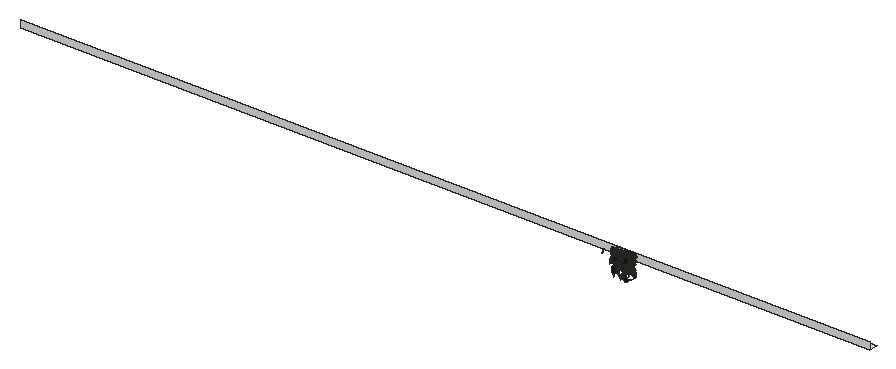
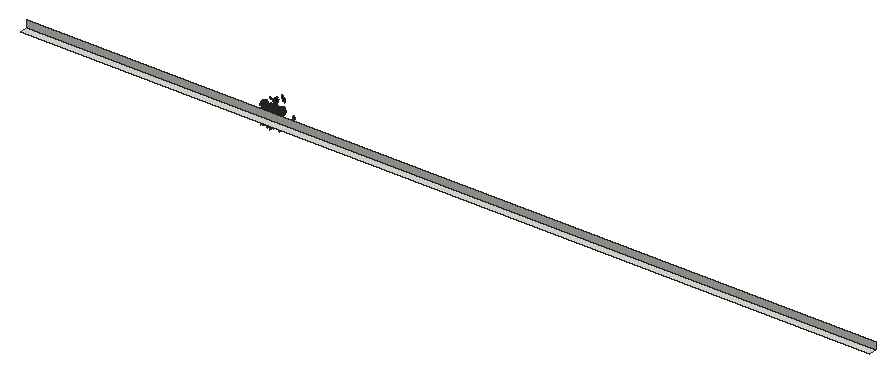
# SketchUp Ruby script. Lengths in inches.
U = 1.inch
M = Sketchup.active_model
def pt(a) = Geom::Point3d.new(a.map { |v| v * U })
def face(e, loops, mat)
  f = e.add_face(loops[0].map { |a| pt(a) })
  loops[1..].each { |l| e.add_face(l.map { |a| pt(a) }).erase! }
  f.material = f.back_material = mat if mat
  f
end
# faces: each face lists its corners as indices into pts; further lists are holes
def faces(e, pts, list, mat = nil) = list.each { |f| face(e, (f[0].is_a?(Array) ? f : [f]).map { |l| l.map { |i| pts[i] } }, mat) }
# xy, xz, yz: faces in a plane at the given z, y or x. An outline is a flat list of corners, or four numbers for a rectangle; further outlines are holes
def ring(l) = l.size == 4 ? [[l[0], l[1]], [l[2], l[1]], [l[2], l[3]], [l[0], l[3]]] : l.each_slice(2).to_a
def flat(e, list, mat, &to3) = list.each { |f| face(e, (f[0].is_a?(Array) ? f : [f]).map { |l| ring(l).map { |u, v| to3.(u, v) } }, mat) }
def xy(e, z, list, mat = nil) = flat(e, list, mat) { |x, y| [x, y, z] }
def xz(e, y, list, mat = nil) = flat(e, list, mat) { |x, z| [x, y, z] }
def yz(e, x, list, mat = nil) = flat(e, list, mat) { |y, z| [x, y, z] }
def lines(e, pts, list) = list.each { |a, b| e.add_line(pt(pts[a]), pt(pts[b])) }
# prism: a flat outline (further loops are holes) pulled along v
def prism(e, loops, v, mat = nil)
  f = face(e, loops, mat); d = Geom::Vector3d.new(v.map { |x| x * U })
  f.pushpull(f.normal.samedirection?(d) ? d.length : -d.length)
end
def box(e, o, s, mat = nil) = prism(e, [[o, [o[0] + s[0], o[1], o[2]], [o[0] + s[0], o[1] + s[1], o[2]], [o[0], o[1] + s[1], o[2]]]], [0, 0, s[2]], mat)
def at(x, y, z, deg = 0) = Geom::Transformation.translation(pt([x, y, z])) * Geom::Transformation.rotation(ORIGIN, Z_AXIS, deg.degrees)
def axes(o, x, y, z) = Geom::Transformation.new([*x, 0, *y, 0, *z, 0, *pt(o).to_a, 1])
def part(name) = M.definitions.add(name)
# library, detail: a bought-in or finely detailed component or shape, given as its bounding box
def library(name, o, s) = part(name).tap { |d| box(d.entities, o, s) }
def detail(e, o, s) = box(e.add_group.entities, o, s)
def put(e, d, t, mat = nil) = e.add_instance(d, t).tap { |i| i.material = mat if mat }
def group(e, t, mat = nil) = e.add_group.tap { |g| g.transformation = t; g.material = mat if mat }.entities
root = M.entities
M.materials.add("efeu1").color = [18, 25, 13]
M.materials.add("efeu2").color = [43, 57, 29]
c1 = part("ivyleaf_10")
p = [[0,0.5,-0.03],[-0.0625,2.02,-0.43],[-0.19,2.01,-0.46],[-0.54,1.05,-0.29],[-0.52,0.625,-0.18],[-0.83,0.76,-0.28],
  [-1.16,0.64,-0.33],[-1.15,0.33,-0.24],[-0.77,-0.39,0.02],[-0.3,-0.51,0.16],[0.04,-0.48,0.23],[-0.02,2.01,-0.4375],
  [-0.06,2.01,-0.43],[0.04,-0.49,0.23],[0.67,-0.49,0.14],[1.38,0.36,-0.2],[1.375,0.51,-0.24],[0.81,0.65,-0.19],
  [0.62,0.59,-0.15],[0.6,1.09,-0.28],[0.5,1.23,-0.31]]
faces(c1.entities,p,[[0,1,2,3,4,5,6,7,8,9,10],[11,12,0,13,14,15,16,17,18,19,20]],"efeu2")
c2 = part("ivyleaf_9")
p = [[1.54,2.16,1.25],[1.36,2.04,1.19],[-0.21,0.99,0.68],[-0.71,1.11,0.82],[-0.85,0.86,0.67],[-0.8,0.17,0.21],
  [-0.9,-0.01,0.1],[-0.67,-0.16,-0.02],[-0.08,-0.08,-0.05],[-0.03,-0.6,-0.4],[0.65,-0.88,-0.66],[0.83,-0.6,-0.49],
  [1.29,-0.42,-0.43],[1.8125,-0.07,-0.26],[1.21,0.44,0.15]]
faces(c2.entities,p,[[0,1,2,3,4,5,6,7,8,9,10,11,12,13,14]],"efeu1")
xy(root,168.16,[[244.16,136.53,244.11,139.97,600.44,145.72,600.49,142.28]])
p = [[244.16,136.53,171.1],[244.16,136.53,168.16],[600.49,142.28,168.16],[600.49,142.28,171.1]]
faces(root,p,[[0,1,2,3]])
put(root,c1,axes([491.37,136.93,169.94],[0.20074,-0.58166,-0.17189],[-0.07454,0.15603,-0.61504],[0.60193,0.2133,-0.01884]))
put(root,c1,axes([494.35,138.04,166.5],[-0.38169,-0.3296,0.38813],[-0.23509,-0.31621,-0.49971],[0.45167,-0.44311,0.0679]))
put(root,c1,axes([494.3,137.58,168],[0.18373,-0.60834,0.06607],[0.02662,-0.06098,-0.63543],[0.61134,0.18548,0.00781]))
put(root,c1,axes([494.72,137.03,171.04],[-0.16372,0.54731,0.35458],[-0.09874,0.34056,-0.57127],[-0.64461,-0.19117,-0.00256]))
put(root,c1,axes([495.41,137.17,171.99],[-0.50295,0.27441,0.28094],[-0.23738,0.15124,-0.57268],[-0.31286,-0.55589,-0.01712]))
put(root,c1,axes([495.4,138.16,164.79],[-0.06945,-0.30835,0.55556],[0.2111,-0.53832,-0.27239],[0.5993,0.15389,0.16033]))
put(root,c1,axes([495.74,137.63,167.37],[-0.02299,0.08652,0.64605],[-0.24024,-0.60207,0.07208],[0.60593,-0.23542,0.05309]))
put(root,c1,axes([495.42,137.59,171.71],[0.40154,0.35078,0.36417],[0.24129,0.27573,-0.53165],[-0.44435,0.46672,0.04039]))
put(root,c1,axes([495.91,137.89,166.02],[-0.33828,0.54486,-0.11963],[-0.06404,0.10105,0.64133],[0.55415,0.34429,0.00109]))
put(root,c1,axes([495.81,138.47,171.13],[0.42104,0.45198,-0.16049],[-0.13431,-0.09391,-0.61682],[-0.46044,0.44069,0.03316]))
put(root,c1,axes([495.91,138.46,171.92],[-0.42511,-0.46934,-0.09728],[0.07791,0.06064,-0.63302],[0.47294,-0.43186,0.01684]))
put(root,c1,axes([496.16,136.59,170.65],[-0.30939,0.56323,-0.31644],[-0.21372,0.24187,0.63946],[0.60966,0.37062,0.06358]))
put(root,c1,axes([495.99,137.91,167.24],[-0.27662,-0.55222,-0.22368],[0.11697,0.19147,-0.61738],[0.5842,-0.29982,0.0177]))
put(root,c1,axes([496.46,136.32,171.12],[0.49785,0.21772,0.48822],[-0.49567,-0.06182,0.53302],[0.20018,-0.69455,0.1056]))
put(root,c1,axes([496.28,138.06,165.92],[-0.42104,-0.49881,-0.03379],[0.02216,0.02551,-0.65276],[0.49947,-0.42162,0.00047]))
put(root,c1,axes([496.07,137.51,168],[0.35036,-0.44946,-0.33138],[0.21257,-0.25441,0.5698],[-0.51638,-0.40969,0.00971]))
put(root,c1,axes([496.4,136.3125,170.78],[0.10647,0.40993,-0.5934],[-0.19201,-0.56207,-0.42274],[-0.69519,0.21803,0.02588]))
put(root,c1,axes([496.23,137.45,168.42],[-0.01041,-0.29068,-0.5946],[0.25253,0.54794,-0.27229],[0.61178,-0.23112,0.10228]))
put(root,c1,axes([496.05,138.15,165.57],[0.10042,-0.21579,0.59118],[0.49955,-0.33678,-0.20779],[0.38277,0.49614,0.11608]))
put(root,c1,axes([496.48,138.45,171.625],[0.40132,-0.46532,-0.1728],[-0.02022,0.2067,-0.60357],[0.49595,0.38495,0.11522]))
put(root,c1,axes([496.59,137.33,163.82],[-0.26189,0.61671,-0.02893],[-0.02972,0.0188,0.66972],[0.61667,0.26281,0.01999]))
put(root,c1,axes([496.76,137.29,171.625],[-0.1186,-0.41896,0.51867],[-0.09612,-0.51056,-0.4344],[0.65978,-0.14969,0.02994]))
put(root,c1,axes([496.72,137.96,167.28],[0.38216,-0.48918,-0.19687],[-0.07454,0.19057,-0.61824],[0.52201,0.38533,0.05584]))
put(root,c1,axes([496.74,138.22,166.36],[0.05447,-0.62598,0.15616],[0.00519,-0.15628,-0.6283],[0.64515,0.05411,-0.00814]))
put(root,c1,axes([496.53,137.5,164.18],[-0.42838,0.39711,-0.32232],[0.23428,-0.22138,-0.58412],[-0.45464,-0.48825,0.00269]))
put(root,c1,axes([496.64,137.7,169.19],[-0.54602,-0.15423,-0.35911],[0.34067,0.11457,-0.56718],[0.19155,-0.6434,-0.01491]))
put(root,c1,axes([496.97,138.02,166.98],[-0.07813,-0.47329,0.43932],[0.21012,-0.43708,-0.4335],[0.61062,0.08984,0.20539]))
put(root,c1,axes([497.31,137.44,170.81],[-0.10195,-0.54483,-0.38034],[0.05365,0.37679,-0.55412],[0.66228,-0.11439,-0.01366]))
put(root,c1,axes([497.29,138.17,171.52],[0.6453,-0.01167,0.17544],[0.17517,-0.01503,-0.64531],[0.0152,0.66856,-0.01145]))
put(root,c1,axes([497.16,137.5,171.59],[0.44872,0.01675,0.51547],[0.49127,0.1941,-0.43396],[-0.15698,0.65528,0.11537]))
put(root,c2,axes([497.875,135.72,169.93],[-0.00857,0.34709,-0.68068],[-0.05875,-0.679,-0.3455],[-0.7618,0.04846,0.03431]))
put(root,c1,axes([498.13,138.36,172.02],[0.40905,-0.43948,-0.31281],[-0.10873,0.31734,-0.58803],[0.52837,0.40554,0.12116]))
put(root,c1,axes([498.09,137.79,167.62],[0.24899,-0.57995,0.20296],[0.08723,-0.1834,-0.6311],[0.60821,0.26373,0.00743]))
put(root,c1,axes([498.41,137.69,171.96],[0.18426,-0.59688,-0.22796],[-0.03184,0.22837,-0.62371],[0.63814,0.18375,0.0347]))
put(root,c1,axes([498.53,138.64,169.75],[0.09132,-0.5851,-0.3012],[0.04809,0.30921,-0.58608],[0.65632,0.05876,0.08485]))
put(root,c1,axes([498.66,137.7,170.31],[0.21708,-0.5912,0.09438],[0.0354,-0.08754,-0.62979],[0.59764,0.21993,0.00302]))
put(root,c1,axes([499.04,136.47,170.78],[-0.71186,-0.03864,0.11786],[-0.11762,-0.00767,-0.71291],[0.03938,-0.72151,0.00127]))
put(root,c1,axes([498.93,138.17,171.5625],[0.00827,-0.59983,-0.22154],[0.03241,0.22167,-0.59896],[0.63861,-0.00348,0.03327]))
put(root,c1,axes([499.04,137.17,172.34],[0.15338,0.48706,-0.49016],[-0.27108,-0.41944,-0.50161],[-0.63562,0.29641,0.09564]))
put(root,c1,axes([499.08,137.56,170.8125],[-0.27495,-0.45174,0.43415],[-0.01275,-0.46998,-0.4971],[0.62641,-0.20785,0.18044]))
put(root,c2,axes([498.57,135.99,164.49],[0.33118,-0.63402,0.25519],[0.14752,-0.21058,-0.71462],[0.66734,0.3612,0.03132]))
put(root,c1,axes([499.12,138.23,168.7],[0.05039,-0.56776,-0.30934],[-0.0266,0.30819,-0.57],[0.64602,0.05698,0.00066]))
put(root,c1,axes([499.15,138.19,171.27],[-0.08401,-0.60914,-0.1781],[0.02614,0.17618,-0.6149],[0.6341,-0.08797,0.00175]))
put(root,c1,axes([499.37,135.59,166.78],[-0.70892,-0.00909,0.18833],[-0.18787,-0.02782,-0.70856],[0.01592,-0.73299,0.02456]))
put(root,c1,axes([499.44,136.58,170.88],[0.07467,-0.36935,-0.6145],[-0.0391,0.61481,-0.37429],[0.71589,0.0721,0.04365]))
put(root,c1,axes([499.08,136.76,169.66],[0.63463,-0.03986,-0.32095],[0.3222,0.0167,0.63503],[-0.02801,-0.71097,0.03291]))
put(root,c1,axes([499.6,138.25,172.07],[-0.07345,-0.5592,0.29973],[0.02693,-0.30421,-0.56096],[0.63389,-0.05187,0.05856]))
put(root,c1,axes([499.58,138.42,164.26],[-0.4626,-0.35241,-0.27711],[0.21764,0.17158,-0.58153],[0.39194,-0.51122,-0.00415]))
put(root,c2,axes([499.17,135.22,169.24],[0.44522,-0.57903,0.296],[0.17857,-0.23607,-0.73041],[0.6253,0.4797,-0.00216]))
put(root,c1,axes([499.6,138.1,171.76],[0.09958,-0.19788,0.61403],[0.41408,-0.45682,-0.21437],[0.4947,0.42221,0.05584]))
put(root,c1,axes([500.26,138.51,171.95],[-0.30746,0.5382,0.14897],[-0.07256,0.13012,-0.61983],[-0.5537,-0.3159,-0.0015]))
put(root,c1,axes([499.93,138.07,171.49],[0.27514,-0.17693,0.57143],[0.52844,-0.22289,-0.32345],[0.28035,0.59377,0.04886]))
put(root,c1,axes([500.47,137.58,171.32],[0.06377,-0.60765,0.19177],[0.05217,-0.1871,-0.6102],[0.63505,0.07639,0.03087]))
put(root,c1,axes([500.56,138.22,171.99],[-0.06747,-0.58687,0.25621],[0.00709,-0.25829,-0.58978],[0.64032,-0.05897,0.03353]))
put(root,c1,axes([500.38,137.72,170.71],[-0.551,0.25416,-0.27255],[0.23552,-0.13951,-0.60625],[-0.28881,-0.59868,0.02557]))
put(root,c1,axes([500.92,138.3,165.125],[0.39825,0.12397,-0.51768],[-0.5065,-0.11064,-0.41615],[-0.16376,0.6437,0.02817]))
put(root,c1,axes([500.99,134.75,169.85],[-0.19122,0.4073,-0.62117],[-0.27142,0.55876,0.44993],[0.69143,0.33198,0.00483]))
put(root,c1,axes([500.51,137.7,166.81],[-0.16655,-0.21523,0.6372],[0.36962,0.51913,0.27196],[-0.56189,0.40529,-0.00997]))
put(root,c1,axes([500.92,137.24,171.79],[0.23584,-0.47733,-0.38288],[-0.01489,0.40573,-0.515],[0.61173,0.1939,0.13507]))
put(root,c1,axes([500.9375,137.82,170.98],[0.29972,-0.5147,-0.24679],[-0.046,0.25606,-0.58989],[0.56896,0.29184,0.08232]))
put(root,c2,axes([500.32,135.43,167.79],[0.53431,0.13221,-0.57329],[0.54692,0.17381,0.54982],[0.21684,-0.76416,0.02587]))
put(root,c1,axes([501.05,137.46,168.99],[0.09058,-0.27183,0.6442],[0.17401,-0.62038,-0.28625],[0.6772,0.19577,-0.01261]))
put(root,c1,axes([501.01,138.47,167.15],[-0.34183,0.50423,-0.18434],[0.10268,-0.15309,-0.60918],[-0.52696,-0.35692,0.00088]))
put(root,c1,axes([501.61,138.69,167.39],[-0.00767,0.03151,-0.64129],[-0.60473,0.21513,0.0178],[0.21573,0.60417,0.0271]))
put(root,c2,axes([501.0625,135.32,168.37],[0.22671,-0.72111,-0.27887],[-0.07101,0.26997,-0.75581],[0.76989,0.23725,0.01241]))
put(root,c1,axes([501.54,138.13,171.81],[0.54534,0.11754,-0.33467],[-0.33667,-0.0217,-0.55624],[-0.11166,0.63948,0.04264]))
put(root,c1,axes([501.48,134.64,169.32],[0.3941,-0.66968,0.01112],[0.00564,-0.00958,-0.77704],[0.66975,0.39414,0]))
put(root,c1,axes([501.17,135.54,167.04],[0.47766,-0.34629,0.5412],[0.4369,-0.3194,-0.58998],[0.4711,0.64733,-0.00159]))
put(root,c1,axes([501.69,137.79,164.02],[-0.00284,-0.01683,-0.71011],[-0.13179,0.6978,-0.01601],[0.69798,0.13168,-0.00592]))
put(root,c1,axes([501.91,138.39,166.15],[-0.12527,0.16685,-0.62025],[-0.42195,0.45507,0.20764],[0.48426,0.43968,0.02047]))
put(root,c1,axes([501.61,138.1,166.76],[0.06302,-0.05618,0.67062],[-0.16562,0.65154,0.07015],[-0.65227,-0.17086,0.04699]))
put(root,c1,axes([501.24,136.98,165.625],[0.43171,-0.31501,-0.50248],[0.39139,-0.3156,0.53413],[-0.44556,-0.58245,-0.01767]))
put(root,c1,axes([501.6875,138.01,170.68],[-0.40615,-0.4384,-0.2488],[0.19345,0.15949,-0.59682],[0.46548,-0.4488,0.03094]))
put(root,c1,axes([501.56,138.45,167.36],[-0.48104,0.0488,-0.42972],[0.42691,-0.0493,-0.48348],[-0.06922,-0.64314,0.00446]))
put(root,c1,axes([502.31,138.18,171.46],[0.12757,0.19016,-0.60358],[-0.6145,0.18432,-0.07181],[0.15118,0.58873,0.21744]))
put(root,c1,axes([501.625,136.91,165.375],[0.12539,-0.16207,0.709],[0.3806,-0.59846,-0.20411],[0.61975,0.40031,-0.0181]))
put(root,c1,axes([502.37,138.46,169.18],[-0.16464,0.16467,-0.61021],[-0.63079,-0.00309,0.16936],[0.03981,0.63203,0.15982]))
put(root,c1,axes([502.03,137.86,171.75],[0.18101,-0.48184,-0.40156],[-0.04349,0.4073,-0.50833],[0.62572,0.1677,0.08083]))
put(root,c1,axes([501.9,135.43,165.9],[-0.67489,-0.37921,0.22381],[0.19855,0.10352,0.77411],[-0.39303,0.70346,0.00674]))
put(root,c1,axes([502.41,138.22,167.32],[0.33057,-0.04984,-0.57145],[-0.56489,0.08633,-0.3343],[0.09968,0.65451,0.00058]))
put(root,c1,axes([502.14,138.08,169.99],[0.60782,0.14069,-0.19865],[-0.19671,-0.03088,-0.62374],[-0.1434,0.63871,0.0136]))
put(root,c1,axes([502.36,137.77,169.27],[0.1123,-0.02585,-0.67985],[0.05513,0.68713,-0.01702],[0.6781,-0.05158,0.11398]))
put(root,c1,axes([502.14,138.31,165.27],[0.2461,-0.34978,0.49712],[0.31202,-0.38757,-0.42716],[0.52164,0.39684,0.02098]))
put(root,c1,axes([502.49,137.21,171.22],[-0.3139,-0.52713,0.19046],[-0.04695,-0.1928,-0.61098],[0.55851,-0.31247,0.05569]))
put(root,c1,axes([502.42,137.83,169.23],[0.09711,-0.57688,0.26469],[0.02302,-0.2644,-0.58468],[0.63429,0.09792,-0.01931]))
put(root,c1,axes([502.73,138.04,168.5625],[0.42085,-0.16994,-0.48499],[-0.45141,0.17735,-0.45386],[0.24561,0.61716,-0.00312]))
put(root,c2,axes([502.18,136.23,170.17],[0.204,-0.66947,-0.30407],[-0.06322,0.29841,-0.69944],[0.73257,0.21219,0.02431]))
put(root,c2,axes([502.15,129.01,170.32],[-0.53426,-0.00789,-0.83358],[0.86561,0.00689,-0.51452],[0.01081,-0.94186,0.00322]))
put(root,c1,axes([502.35,138.3,170.44],[-0.54078,0.16487,-0.30269],[0.28248,-0.11071,-0.56498],[-0.19751,-0.60976,0.02074]))
put(root,c1,axes([502.09,137.53,171.41],[0.1865,-0.17478,0.66487],[0.63343,-0.22402,-0.23657],[0.26715,0.65318,0.09677]))
put(root,c1,axes([502.48,138.39,166.43],[-0.53745,-0.21297,-0.30948],[0.28199,0.12822,-0.57795],[0.24822,-0.60679,-0.0135]))
put(root,c1,axes([502.52,138.33,171.86],[-0.3183,-0.35708,-0.43601],[0.35581,0.261,-0.4735],[0.43705,-0.47255,0.06795]))
put(root,c1,axes([502.79,137.8,166.66],[-0.0985,-0.50468,0.37459],[0.08199,-0.38624,-0.49882],[0.62314,-0.02895,0.12484]))
put(root,c1,axes([502.99,137.97,170.99],[-0.29661,-0.47972,0.32499],[-0.04878,-0.34313,-0.55101],[0.57738,-0.27543,0.12041]))
put(root,c2,axes([503.48,133.64,171.35],[-0.67329,0.06996,-0.45742],[-0.45676,0.02883,0.67674],[0.07409,0.81346,0.01535]))
put(root,c1,axes([502.83,133.48,165.96],[0.0798,-0.35651,0.71863],[0.24892,-0.67553,-0.36277],[0.76261,0.2578,0.04321]))
put(root,c1,axes([502.71,138.36,165.46],[0.53704,-0.25445,0.29182],[0.27628,-0.09774,-0.59366],[0.27124,0.60334,0.0269]))
put(root,c1,axes([503.19,138.08,171.89],[0.15014,-0.62987,-0.03437],[-0.00594,0.03391,-0.64751],[0.63078,0.15024,0.00209]))
put(root,c1,axes([503.06,138.07,169.92],[-0.00476,-0.59614,-0.30589],[0.08652,-0.30388,0.59089],[-0.66443,-0.0353,0.07913]))
put(root,c1,axes([502.82,138.13,167.27],[0.10098,-0.14159,0.61257],[0.56129,-0.25923,-0.15244],[0.28327,0.56413,0.08369]))
put(root,c1,axes([503.51,138.24,164.8],[0.43747,-0.23475,-0.45474],[-0.40455,0.20776,-0.49644],[0.31342,0.59582,-0.00606]))
put(root,c1,axes([502.86,138.39,164.81],[-0.38692,0.0765,-0.53333],[0.52565,-0.09049,-0.39433],[-0.11823,-0.65265,-0.00784]))
put(root,c1,axes([503.29,138.07,172.06],[0.31163,-0.52045,-0.23254],[-0.04767,0.2403,-0.6017],[0.56804,0.30569,0.07708]))
put(root,c1,axes([503.08,137.05,170.96],[0.32279,-0.50679,-0.23509],[0.14656,-0.18518,0.60043],[-0.5391,-0.35379,0.02248]))
put(root,c2,axes([503.07,131.21,170.05],[0.89502,-0.1137,-0.3368],[-0.34099,0.07934,-0.86926],[0.14536,0.88621,0.03462]))
put(root,c1,axes([503.4375,137.58,170.36],[-0.26054,-0.59721,0.03733],[-0.01239,-0.03533,-0.65156],[0.59824,-0.26082,0.00277]))
put(root,c1,axes([503.51,133.3125,165.27],[0.22292,-0.57055,0.53871],[-0.20237,0.49928,0.61253],[-0.75814,-0.30103,-0.00511]))
put(root,c1,axes([503.55,137.88,169.28],[0.06675,-0.64604,-0.0109],[0.00119,0.01108,-0.64947],[0.64613,0.06672,0.00233]))
put(root,c1,axes([503.21,137.9,166.17],[0.39601,-0.27152,0.42386],[0.37245,-0.20474,-0.47913],[0.33861,0.54274,0.0313]))
put(root,c1,axes([503.33,137.95,169.16],[-0.03975,-0.16741,-0.62246],[0.16205,-0.6062,0.15269],[-0.62387,-0.1468,0.07932]))
put(root,c1,axes([503.55,137.99,171.5625],[0.33929,-0.54433,0.07814],[0.08016,-0.04188,-0.6398],[0.54404,0.34564,0.04553]))
put(root,c1,axes([503.45,137.92,168.43],[0.09961,-0.45209,0.44859],[0.2668,-0.38267,-0.44489],[0.57831,0.25441,0.12798]))
put(root,c1,axes([503.29,138.09,168.89],[0.50837,-0.03834,-0.44472],[0.44622,0.02623,0.50783],[-0.01153,-0.67493,0.045]))
put(root,c1,axes([503.49,138.39,164.39],[0.28646,-0.32214,0.46975],[0.32781,-0.33676,-0.43085],[0.46581,0.4351,0.01432]))
put(root,c1,axes([503.84,137.88,171.98],[-0.1173,-0.63702,0.03551],[0.02124,-0.03998,-0.64712],[0.63765,-0.11585,0.02809]))
put(root,c1,axes([504.01,138.33,164.7],[0.30159,-0.36783,-0.45874],[-0.05696,0.49486,-0.43425],[0.58523,0.23773,0.19414]))
put(root,c1,axes([504.01,136.95,169.87],[0.25868,-0.58764,-0.06946],[-0.02253,0.06597,-0.64203],[0.59131,0.25959,0.00592]))
put(root,c1,axes([503.875,135.33,170.35],[0.68192,-0.19023,0.01699],[-0.01392,0.01334,0.7079],[-0.19048,-0.682,0.0091]))
put(root,c1,axes([504.4,137.05,166.93],[0.41388,0.00667,-0.5406],[-0.54059,0.01472,-0.41369],[0.00763,0.68068,0.01424]))
put(root,c1,axes([503.53,137.02,171.08],[0.2239,-0.11575,-0.69846],[0.68385,-0.15429,0.24479],[-0.18328,-0.71706,0.06008]))
put(root,c1,axes([504,137.25,167.57],[0.14136,-0.72803,-0.09826],[0.03291,-0.09369,0.74149],[-0.73389,-0.14444,0.01433]))
put(root,c1,axes([504.26,137.99,171.4375],[-0.1486,-0.54278,0.31521],[0.09999,-0.34026,-0.53878],[0.61966,-0.07526,0.16252]))
put(root,c2,axes([503.72,133.27,164.7],[0.32561,-0.01227,0.75109],[0.75079,0.0319,-0.32496],[-0.02439,0.81801,0.02394]))
